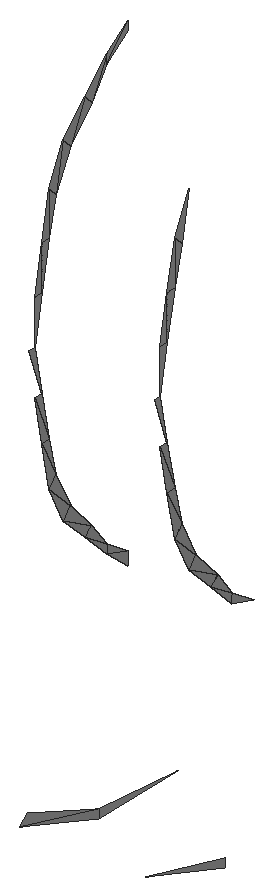
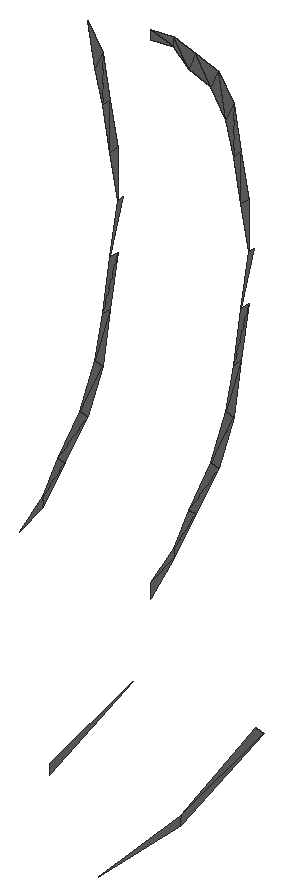
# SketchUp Ruby script. Lengths in inches.
U = 1.inch
M = Sketchup.active_model
def pt(a) = Geom::Point3d.new(a.map { |v| v * U })
def face(e, loops, mat)
  f = e.add_face(loops[0].map { |a| pt(a) })
  loops[1..].each { |l| e.add_face(l.map { |a| pt(a) }).erase! }
  f.material = f.back_material = mat if mat
  f
end
# faces: each face lists its corners as indices into pts; further lists are holes
def faces(e, pts, list, mat = nil) = list.each { |f| face(e, (f[0].is_a?(Array) ? f : [f]).map { |l| l.map { |i| pts[i] } }, mat) }
# xy, xz, yz: faces in a plane at the given z, y or x. An outline is a flat list of corners, or four numbers for a rectangle; further outlines are holes
def ring(l) = l.size == 4 ? [[l[0], l[1]], [l[2], l[1]], [l[2], l[3]], [l[0], l[3]]] : l.each_slice(2).to_a
def flat(e, list, mat, &to3) = list.each { |f| face(e, (f[0].is_a?(Array) ? f : [f]).map { |l| ring(l).map { |u, v| to3.(u, v) } }, mat) }
def xy(e, z, list, mat = nil) = flat(e, list, mat) { |x, y| [x, y, z] }
def xz(e, y, list, mat = nil) = flat(e, list, mat) { |x, z| [x, y, z] }
def yz(e, x, list, mat = nil) = flat(e, list, mat) { |y, z| [x, y, z] }
def lines(e, pts, list) = list.each { |a, b| e.add_line(pt(pts[a]), pt(pts[b])) }
# prism: a flat outline (further loops are holes) pulled along v
def prism(e, loops, v, mat = nil)
  f = face(e, loops, mat); d = Geom::Vector3d.new(v.map { |x| x * U })
  f.pushpull(f.normal.samedirection?(d) ? d.length : -d.length)
end
def box(e, o, s, mat = nil) = prism(e, [[o, [o[0] + s[0], o[1], o[2]], [o[0] + s[0], o[1] + s[1], o[2]], [o[0], o[1] + s[1], o[2]]]], [0, 0, s[2]], mat)
def at(x, y, z, deg = 0) = Geom::Transformation.translation(pt([x, y, z])) * Geom::Transformation.rotation(ORIGIN, Z_AXIS, deg.degrees)
def axes(o, x, y, z) = Geom::Transformation.new([*x, 0, *y, 0, *z, 0, *pt(o).to_a, 1])
def part(name) = M.definitions.add(name)
# library, detail: a bought-in or finely detailed component or shape, given as its bounding box
def library(name, o, s) = part(name).tap { |d| box(d.entities, o, s) }
def detail(e, o, s) = box(e.add_group.entities, o, s)
def put(e, d, t, mat = nil) = e.add_instance(d, t).tap { |i| i.material = mat if mat }
def group(e, t, mat = nil) = e.add_group.tap { |g| g.transformation = t; g.material = mat if mat }.entities
root = M.entities
M.materials.add("Material \#1").color = [140, 140, 140]
yz(root,155.64,[[443.91,49.89,443.91,49.9,443.8,49.93],[443.91,49.89,444.02,49.89,443.91,49.9],[443.91,49.9,443.81,49.94,443.8,49.93],[443.95,50.125,443.95,50.14,443.92,50.15],[443.95,50.14,443.92,50.16,443.92,50.15],
  [443.92,50.15,443.92,50.16,443.89,50.18],[443.92,50.16,443.9,50.1875,443.89,50.18],[443.89,50.18,443.9,50.1875,443.86,50.21],[443.9,50.1875,443.87,50.22,443.86,50.21],[443.86,50.21,443.87,50.22,443.84,50.25],
  [443.87,50.22,443.85,50.26,443.84,50.25],[443.84,50.25,443.85,50.26,443.83,50.3],[443.85,50.26,443.84,50.3,443.83,50.3],[443.83,50.3,443.84,50.3,443.82,50.35],[443.84,50.3,443.83,50.35,443.82,50.35],
  [443.83,50.35,443.82,50.4,443.8125,50.4],[443.82,50.4,443.83,50.45,443.82,50.45],[443.82,50.45,443.83,50.45,443.83,50.5],[443.83,50.45,443.84,50.5,443.83,50.5],[443.83,50.5,443.84,50.5,443.84,50.55],
  [443.84,50.5,443.85,50.54,443.84,50.55],[443.85,50.54,443.86,50.59,443.84,50.55],[443.85,50.54,443.87,50.58,443.86,50.59],[443.87,50.58,443.89,50.62,443.86,50.59],[443.87,50.58,443.9,50.61,443.89,50.62],
  [443.9,50.61,443.92,50.65,443.89,50.62],[443.9,50.61,443.92,50.64,443.92,50.65],[443.92,50.64,443.95,50.66,443.95,50.67],[443.92,50.64,443.95,50.67,443.92,50.65]],"Material \#1")
yz(root,155.78,[[443.91,49.89,443.8,49.93,443.91,49.9],[443.95,50.14,443.92,50.15,443.92,50.16],[443.92,50.15,443.89,50.18,443.92,50.16],[443.92,50.16,443.89,50.18,443.9,50.1875],[443.89,50.18,443.86,50.21,443.9,50.1875],
  [443.9,50.1875,443.86,50.21,443.87,50.22],[443.86,50.21,443.84,50.25,443.87,50.22],[443.87,50.22,443.84,50.25,443.85,50.26],[443.84,50.25,443.83,50.3,443.85,50.26],[443.85,50.26,443.83,50.3,443.84,50.3],
  [443.83,50.3,443.82,50.35,443.84,50.3],[443.84,50.3,443.82,50.35,443.83,50.35],[443.83,50.35,443.8125,50.4,443.82,50.4],[443.82,50.4,443.82,50.45,443.83,50.45],[443.82,50.45,443.83,50.5,443.83,50.45],
  [443.83,50.45,443.83,50.5,443.84,50.5],[443.83,50.5,443.84,50.55,443.84,50.5],[443.84,50.5,443.84,50.55,443.85,50.54],[443.85,50.54,443.84,50.55,443.86,50.59]],"Material \#1")
